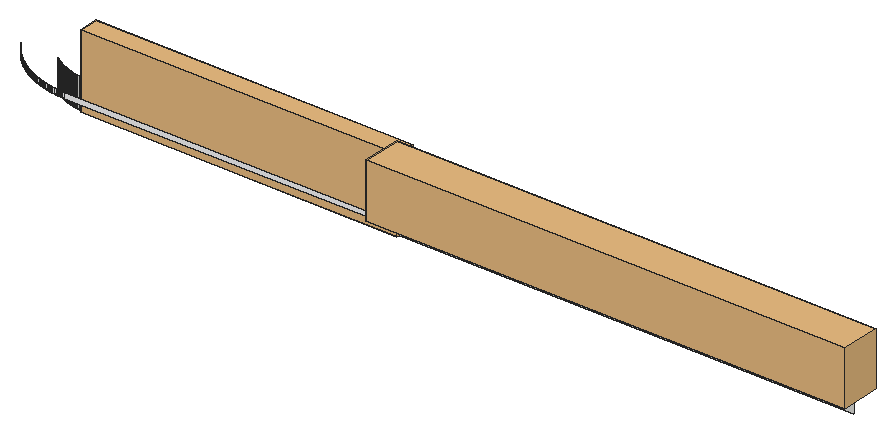
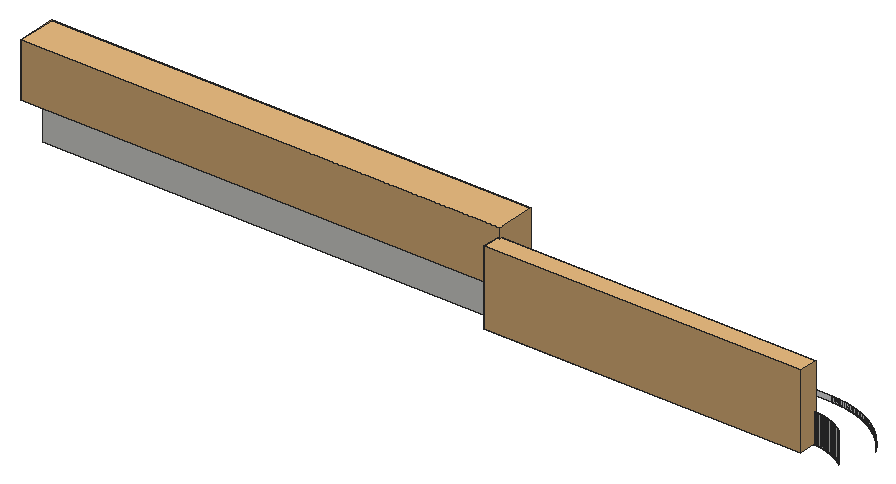
# SketchUp Ruby script. Lengths in inches.
U = 1.inch
M = Sketchup.active_model
def pt(a) = Geom::Point3d.new(a.map { |v| v * U })
def face(e, loops, mat)
  f = e.add_face(loops[0].map { |a| pt(a) })
  loops[1..].each { |l| e.add_face(l.map { |a| pt(a) }).erase! }
  f.material = f.back_material = mat if mat
  f
end
# faces: each face lists its corners as indices into pts; further lists are holes
def faces(e, pts, list, mat = nil) = list.each { |f| face(e, (f[0].is_a?(Array) ? f : [f]).map { |l| l.map { |i| pts[i] } }, mat) }
# xy, xz, yz: faces in a plane at the given z, y or x. An outline is a flat list of corners, or four numbers for a rectangle; further outlines are holes
def ring(l) = l.size == 4 ? [[l[0], l[1]], [l[2], l[1]], [l[2], l[3]], [l[0], l[3]]] : l.each_slice(2).to_a
def flat(e, list, mat, &to3) = list.each { |f| face(e, (f[0].is_a?(Array) ? f : [f]).map { |l| ring(l).map { |u, v| to3.(u, v) } }, mat) }
def xy(e, z, list, mat = nil) = flat(e, list, mat) { |x, y| [x, y, z] }
def xz(e, y, list, mat = nil) = flat(e, list, mat) { |x, z| [x, y, z] }
def yz(e, x, list, mat = nil) = flat(e, list, mat) { |y, z| [x, y, z] }
def lines(e, pts, list) = list.each { |a, b| e.add_line(pt(pts[a]), pt(pts[b])) }
# prism: a flat outline (further loops are holes) pulled along v
def prism(e, loops, v, mat = nil)
  f = face(e, loops, mat); d = Geom::Vector3d.new(v.map { |x| x * U })
  f.pushpull(f.normal.samedirection?(d) ? d.length : -d.length)
end
def box(e, o, s, mat = nil) = prism(e, [[o, [o[0] + s[0], o[1], o[2]], [o[0] + s[0], o[1] + s[1], o[2]], [o[0], o[1] + s[1], o[2]]]], [0, 0, s[2]], mat)
def at(x, y, z, deg = 0) = Geom::Transformation.translation(pt([x, y, z])) * Geom::Transformation.rotation(ORIGIN, Z_AXIS, deg.degrees)
def axes(o, x, y, z) = Geom::Transformation.new([*x, 0, *y, 0, *z, 0, *pt(o).to_a, 1])
def part(name) = M.definitions.add(name)
# library, detail: a bought-in or finely detailed component or shape, given as its bounding box
def library(name, o, s) = part(name).tap { |d| box(d.entities, o, s) }
def detail(e, o, s) = box(e.add_group.entities, o, s)
def put(e, d, t, mat = nil) = e.add_instance(d, t).tap { |i| i.material = mat if mat }
def group(e, t, mat = nil) = e.add_group.tap { |g| g.transformation = t; g.material = mat if mat }.entities
root = M.entities
M.materials.add("[Quartz Light Grey]").color = [251, 251, 252]
M.materials.add("[Wood Cherry Original]1").color = [176, 123, 88]
c1 = library("Group\#14",[0,-5,0],[194.81,16,22])
c2 = library("Group\#15",[67,-1,0],[128.81,8,30])
xz(root,151,[[44.67,297.82,45,299.82],[45,297.82,171.19,299.82]],"[Quartz Light Grey]")
xz(root,151.01,[[44.01,297.82,44.34,299.82]],"[Quartz Light Grey]")
xz(root,162,[[44.53,287.82,44.76,299.82],[44.76,287.82,45,299.82],[45,287.82,357,299.82]])
yz(root,171.19,[[151,297.82,156,299.82]])
p = [[43.59,162.04,287.82],[43.35,162.05,287.82],[43.35,162.05,299.82],[43.59,162.04,299.82],[43.82,162.03,287.82],[43.82,162.03,299.82],
  [44.06,162.02,287.82],[44.06,162.02,299.82],[44.29,162.01,287.82],[44.29,162.01,299.82],[44.53,162,287.82],[44.53,162,299.82],
  [42.18,162.15,287.82],[41.94,162.17,287.82],[41.94,162.17,299.82],[42.18,162.15,299.82],[42.41,162.125,287.82],[42.41,162.125,299.82],
  [42.65,162.1,287.82],[42.65,162.1,299.82],[42.88,162.08,287.82],[42.88,162.08,299.82],[43.12,162.07,287.82],[43.12,162.07,299.82],
  [41.48,162.23,287.82],[41.24,162.26,287.82],[41.24,162.26,299.82],[41.48,162.23,299.82],[41.71,162.2,287.82],[41.71,162.2,299.82],
  [40.78,162.33,287.82],[40.54,162.37,287.82],[40.54,162.37,299.82],[40.78,162.33,299.82],[41.01,162.3,287.82],[41.01,162.3,299.82],
  [40.3125,162.41,287.82],[40.08,162.45,287.82],[40.08,162.45,299.82],[40.3125,162.41,299.82],[39.62,162.54,287.82],[39.39,162.59,287.82],
  [39.39,162.59,299.82],[39.62,162.54,299.82],[39.85,162.5,287.82],[39.85,162.5,299.82],[39.16,162.64,287.82],[38.93,162.69,287.82],
  [38.93,162.69,299.82],[39.16,162.64,299.82],[38.7,162.75,287.82],[38.47,162.8,287.82],[38.47,162.8,299.82],[38.7,162.75,299.82],
  [38.24,162.86,287.82],[38.24,162.86,299.82],[38.01,162.92,287.82],[37.78,162.98,287.82],[37.78,162.98,299.82],[38.01,162.92,299.82],
  [37.56,163.05,287.82],[37.33,163.11,287.82],[37.33,163.11,299.82],[37.56,163.05,299.82],[37.11,163.18,287.82],[37.11,163.18,299.82],
  [36.88,163.25,287.82],[36.66,163.32,287.82],[36.66,163.32,299.82],[36.88,163.25,299.82],[36.43,163.4,287.82],[36.43,163.4,299.82],
  [36.21,163.47,287.82],[36.21,163.47,299.82],[35.99,163.55,287.82],[35.77,163.63,287.82],[35.77,163.63,299.82],[35.99,163.55,299.82],
  [35.54,163.71,287.82],[35.54,163.71,299.82],[35.32,163.79,287.82],[35.32,163.79,299.82],[35.1,163.88,287.82],[35.1,163.88,299.82],
  [34.89,163.97,287.82],[34.89,163.97,299.82],[34.67,164.06,287.82],[34.67,164.06,299.82],[34.45,164.15,287.82],[34.23,164.24,287.82],
  [34.23,164.24,299.82],[34.45,164.15,299.82],[34.02,164.33,287.82],[34.02,164.33,299.82],[33.8,164.43,287.82],[33.8,164.43,299.82],
  [33.59,164.53,287.82],[33.59,164.53,299.82],[33.375,164.63,287.82],[33.375,164.63,299.82],[33.16,164.73,287.82],[33.16,164.73,299.82],
  [32.95,164.84,287.82],[32.95,164.84,299.82],[32.74,164.94,287.82],[32.74,164.94,299.82],[32.53,165.05,287.82],[32.53,165.05,299.82],
  [32.32,165.16,287.82],[32.32,165.16,299.82],[32.12,165.27,287.82],[32.12,165.27,299.82],[31.91,165.39,287.82],[31.91,165.39,299.82],
  [31.7,165.5,287.82],[31.7,165.5,299.82],[31.5,165.62,287.82],[31.5,165.62,299.82],[31.3,165.74,287.82],[31.3,165.74,299.82],
  [31.09,165.86,287.82],[31.09,165.86,299.82],[30.89,165.98,287.82],[30.89,165.98,299.82],[30.69,166.1,287.82],[30.69,166.1,299.82],
  [30.49,166.23,287.82],[30.49,166.23,299.82],[30.29,166.36,287.82],[30.29,166.36,299.82],[30.1,166.49,287.82],[30.1,166.49,299.82],
  [29.9,166.62,287.82],[29.9,166.62,299.82],[29.71,166.75,287.82],[29.71,166.75,299.82],[29.51,166.88,287.82],[29.51,166.88,299.82],
  [29.32,167.02,287.82],[29.32,167.02,299.82],[29.13,167.16,287.82],[29.13,167.16,299.82],[28.94,167.3,287.82],[28.94,167.3,299.82],
  [43.01,151.05,299.82],[43.01,151.05,297.82],[43.34,151.04,297.82],[43.34,151.04,299.82],[43.67,151.02,297.82],[43.67,151.02,299.82],
  [44.01,151.01,297.82],[44.01,151.01,299.82],[44.34,151.01,299.82],[44.34,151.01,297.82],[44.67,151,297.82],[44.67,151,299.82],
  [41.36,151.17,299.82],[41.36,151.17,297.82],[41.6875,151.14,297.82],[41.6875,151.14,299.82],[42.02,151.12,297.82],[42.02,151.12,299.82],
  [42.35,151.09,297.82],[42.35,151.09,299.82],[42.68,151.07,297.82],[42.68,151.07,299.82],[40.37,151.28,299.82],[40.37,151.28,297.82],
  [40.7,151.24,297.82],[40.7,151.24,299.82],[41.03,151.21,297.82],[41.03,151.21,299.82],[39.71,151.37,299.82],[39.71,151.37,297.82],
  [40.04,151.33,297.82],[40.04,151.33,299.82],[39.06,151.47,299.82],[39.06,151.47,297.82],[39.38,151.42,297.82],[39.38,151.42,299.82],
  [38.4,151.58,299.82],[38.4,151.58,297.82],[38.73,151.52,297.82],[38.73,151.52,299.82],[37.75,151.7,299.82],[37.75,151.7,297.82],
  [38.08,151.64,297.82],[38.08,151.64,299.82],[37.42,151.76,299.82],[37.42,151.76,297.82],[36.78,151.9,299.82],[36.78,151.9,297.82],
  [37.1,151.83,297.82],[37.1,151.83,299.82],[36.45,151.97,299.82],[36.45,151.97,297.82],[35.81,152.13,299.82],[35.81,152.13,297.82],
  [36.13,152.05,297.82],[36.13,152.05,299.82],[35.49,152.21,299.82],[35.49,152.21,297.82],[35.16,152.29,299.82],[35.16,152.29,297.82],
  [34.84,152.38,299.82],[34.84,152.38,297.82],[34.53,152.47,299.82],[34.53,152.47,297.82],[34.21,152.56,299.82],[34.21,152.56,297.82],
  [33.89,152.66,299.82],[33.89,152.66,297.82],[33.57,152.76,299.82],[33.57,152.76,297.82],[33.26,152.86,299.82],[33.26,152.86,297.82],
  [32.94,152.96,299.82],[32.94,152.96,297.82],[32.63,153.07,299.82],[32.63,153.07,297.82],[32.32,153.18,299.82],[32.32,153.18,297.82],
  [32,153.29,299.82],[32,153.29,297.82],[31.69,153.41,299.82],[31.69,153.41,297.82],[31.38,153.52,299.82],[31.38,153.52,297.82],
  [31.07,153.64,299.82],[31.07,153.64,297.82],[30.76,153.77,299.82],[30.76,153.77,297.82],[30.46,153.89,299.82],[30.46,153.89,297.82],
  [30.15,154.02,299.82],[30.15,154.02,297.82],[29.85,154.15,299.82],[29.85,154.15,297.82],[29.54,154.29,299.82],[29.54,154.29,297.82],
  [29.24,154.42,299.82],[29.24,154.42,297.82],[28.94,154.56,299.82],[28.94,154.56,297.82],[28.64,154.7,299.82],[28.64,154.7,297.82],
  [28.34,154.85,299.82],[28.34,154.85,297.82],[28.04,154.99,299.82],[28.04,154.99,297.82],[27.75,155.14,299.82],[27.75,155.14,297.82],
  [27.45,155.29,299.82],[27.45,155.29,297.82],[27.16,155.45,299.82],[27.16,155.45,297.82],[26.87,155.6,299.82],[26.87,155.6,297.82],
  [26.58,155.76,299.82],[26.58,155.76,297.82],[26.29,155.93,299.82],[26.29,155.93,297.82],[26,156.09,299.82],[26,156.09,297.82],
  [25.71,156.26,299.82],[25.71,156.26,297.82],[25.43,156.43,299.82],[25.43,156.43,297.82],[25.15,156.6,299.82],[25.15,156.6,297.82],
  [24.86,156.77,299.82],[24.86,156.77,297.82],[24.58,156.95,299.82],[24.58,156.95,297.82],[24.3,157.13,299.82],[24.3,157.13,297.82],
  [24.03,157.3125,299.82],[24.03,157.3125,297.82],[23.75,157.5,299.82],[23.75,157.5,297.82],[23.48,157.68,299.82],[23.48,157.68,297.82],
  [23.2,157.87,299.82],[23.2,157.87,297.82],[22.93,158.0625,299.82],[22.93,158.0625,297.82],[22.66,158.26,299.82],[22.66,158.26,297.82],
  [22.4,158.45,299.82],[22.4,158.45,297.82],[22.13,158.65,299.82],[22.13,158.65,297.82],[21.87,158.85,299.82],[21.87,158.85,297.82],
  [21.6,159.06,299.82],[21.6,159.06,297.82],[21.34,159.26,299.82],[21.34,159.26,297.82],[21.09,159.47,299.82],[21.09,159.47,297.82],
  [20.83,159.68,299.82],[20.83,159.68,297.82],[20.57,159.89,299.82],[20.57,159.89,297.82],[20.32,160.1,299.82],[20.32,160.1,297.82],
  [20.07,160.32,299.82],[20.07,160.32,297.82],[19.82,160.54,299.82],[19.82,160.54,297.82],[19.57,160.76,299.82],[19.57,160.76,297.82],
  [19.33,160.98,299.82],[19.33,160.98,297.82],[19.08,161.21,299.82],[19.08,161.21,297.82],[18.84,161.4375,299.82],[18.84,161.4375,297.82],
  [18.6,161.67,299.82],[18.6,161.67,297.82],[18.37,161.9,299.82],[18.37,161.9,297.82],[18.13,162.13,299.82],[18.13,162.13,297.82],
  [17.9,162.37,299.82],[17.9,162.37,297.82],[17.67,162.6,299.82],[17.67,162.6,297.82],[17.4375,162.84,299.82],[17.4375,162.84,297.82],
  [17.21,163.08,299.82],[17.21,163.08,297.82],[16.98,163.33,299.82],[16.98,163.33,297.82],[16.76,163.57,299.82],[16.76,163.57,297.82],
  [16.54,163.82,299.82],[16.54,163.82,297.82],[16.32,164.07,299.82],[16.32,164.07,297.82],[16.1,164.32,299.82],[16.1,164.32,297.82],
  [15.89,164.57,299.82],[15.89,164.57,297.82],[15.68,164.83,299.82],[15.68,164.83,297.82],[15.47,165.09,299.82],[15.47,165.09,297.82],
  [15.26,165.34,299.82],[15.26,165.34,297.82],[15.06,165.6,299.82],[15.06,165.6,297.82],[14.85,165.87,299.82],[14.85,165.87,297.82],
  [14.65,166.13,299.82],[14.65,166.13,297.82],[14.45,166.4,299.82],[14.45,166.4,297.82],[14.26,166.66,299.82],[14.26,166.66,297.82],
  [14.0625,166.93,299.82],[14.0625,166.93,297.82],[13.87,167.2,299.82],[13.87,167.2,297.82],[13.68,167.48,299.82],[13.68,167.48,297.82]]
faces(root,p,[[0,1,2,3],[4,0,3,5],[6,4,5,7],[8,6,7,9],[10,8,9,11],[12,13,14,15],[16,12,15,17],[18,16,17,19],
  [20,18,19,21],[22,20,21,23],[1,22,23,2],[24,25,26,27],[28,24,27,29],[13,28,29,14],[30,31,32,33],[34,30,33,35],
  [25,34,35,26],[36,37,38,39],[31,36,39,32],[40,41,42,43],[44,40,43,45],[37,44,45,38],[46,47,48,49],[41,46,49,42],
  [50,51,52,53],[47,50,53,48],[51,54,55,52],[56,57,58,59],[54,56,59,55],[60,61,62,63],[57,60,63,58],[61,64,65,62],
  [66,67,68,69],[64,66,69,65],[67,70,71,68],[70,72,73,71],[74,75,76,77],[72,74,77,73],[75,78,79,76],[78,80,81,79],
  [80,82,83,81],[82,84,85,83],[84,86,87,85],[88,89,90,91],[86,88,91,87],[89,92,93,90],[92,94,95,93],[94,96,97,95],
  [96,98,99,97],[98,100,101,99],[100,102,103,101],[102,104,105,103],[104,106,107,105],[106,108,109,107],[108,110,111,109],[110,112,113,111],
  [112,114,115,113],[114,116,117,115],[116,118,119,117],[118,120,121,119],[120,122,123,121],[122,124,125,123],[124,126,127,125],[126,128,129,127],
  [128,130,131,129],[130,132,133,131],[132,134,135,133],[134,136,137,135],[136,138,139,137],[138,140,141,139],[140,142,143,141]])
faces(root,p,[[144,145,146,147],[147,146,148,149],[149,148,150,151],[152,153,154,155],[156,157,158,159],[159,158,160,161],[161,160,162,163],[163,162,164,165],
  [165,164,145,144],[166,167,168,169],[169,168,170,171],[171,170,157,156],[172,173,174,175],[175,174,167,166],[176,177,178,179],[179,178,173,172],
  [180,181,182,183],[183,182,177,176],[184,185,186,187],[187,186,181,180],[188,189,185,184],[190,191,192,193],[193,192,189,188],[194,195,191,190],
  [196,197,198,199],[199,198,195,194],[200,201,197,196],[202,203,201,200],[204,205,203,202],[206,207,205,204],[208,209,207,206],[210,211,209,208],
  [212,213,211,210],[214,215,213,212],[216,217,215,214],[218,219,217,216],[220,221,219,218],[222,223,221,220],[224,225,223,222],[226,227,225,224],
  [228,229,227,226],[230,231,229,228],[232,233,231,230],[234,235,233,232],[236,237,235,234],[238,239,237,236],[240,241,239,238],[242,243,241,240],
  [244,245,243,242],[246,247,245,244],[248,249,247,246],[250,251,249,248],[252,253,251,250],[254,255,253,252],[256,257,255,254],[258,259,257,256],
  [260,261,259,258],[262,263,261,260],[264,265,263,262],[266,267,265,264],[268,269,267,266],[270,271,269,268],[272,273,271,270],[274,275,273,272],
  [276,277,275,274],[278,279,277,276],[280,281,279,278],[282,283,281,280],[284,285,283,282],[286,287,285,284],[288,289,287,286],[290,291,289,288],
  [292,293,291,290],[294,295,293,292],[296,297,295,294],[298,299,297,296],[300,301,299,298],[302,303,301,300],[304,305,303,302],[306,307,305,304],
  [308,309,307,306],[310,311,309,308],[312,313,311,310],[314,315,313,312],[316,317,315,314],[318,319,317,316],[320,321,319,318],[322,323,321,320],
  [324,325,323,322],[326,327,325,324],[328,329,327,326],[330,331,329,328],[332,333,331,330],[334,335,333,332],[336,337,335,334],[338,339,337,336],
  [340,341,339,338],[342,343,341,340],[344,345,343,342],[346,347,345,344],[348,349,347,346],[350,351,349,348],[352,353,351,350],[354,355,353,352],
  [356,357,355,354],[358,359,357,356],[360,361,359,358],[362,363,361,360],[364,365,363,362]],"[Quartz Light Grey]")
put(root,c1,at(171.19,151,299.82),"[Wood Cherry Original]1")
put(root,c2,at(-23.81,162,287.82),"[Quartz Light Grey]")
